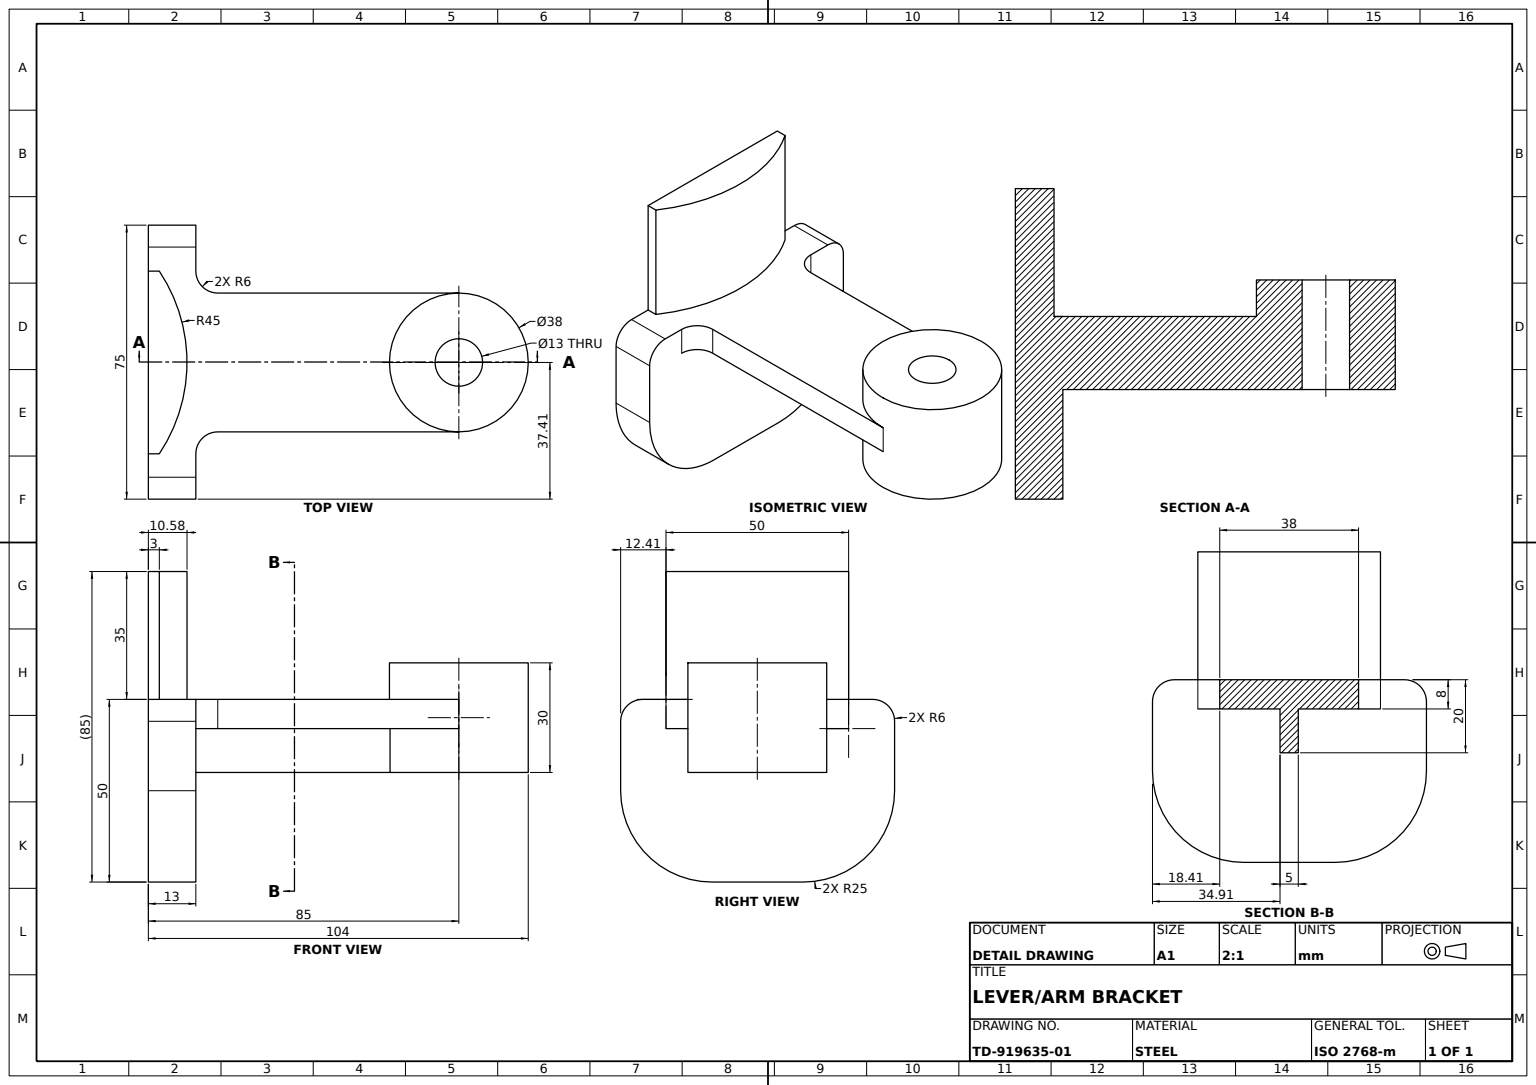
ISO-10303-21;
HEADER;
FILE_DESCRIPTION((''),'2;1');
FILE_NAME('','',(''),(''),'','','');
FILE_SCHEMA(('AUTOMOTIVE_DESIGN'));
ENDSEC;
DATA;
#1=APPLICATION_CONTEXT('');
#2=PRODUCT_CONTEXT('',#1,'mechanical');
#3=PRODUCT('','','',(#2));
#4=PRODUCT_DEFINITION_FORMATION('','',#3);
#5=PRODUCT_DEFINITION_CONTEXT('',#1,'design');
#6=PRODUCT_DEFINITION('','',#4,#5);
#7=PRODUCT_DEFINITION_SHAPE('','',#6);
#8=(LENGTH_UNIT()NAMED_UNIT(*)SI_UNIT(.MILLI.,.METRE.));
#9=(NAMED_UNIT(*)PLANE_ANGLE_UNIT()SI_UNIT($,.RADIAN.));
#10=(NAMED_UNIT(*)SI_UNIT($,.STERADIAN.)SOLID_ANGLE_UNIT());
#11=UNCERTAINTY_MEASURE_WITH_UNIT(LENGTH_MEASURE(1.E-05),#8,'distance_accuracy_value','');
#12=(GEOMETRIC_REPRESENTATION_CONTEXT(3)GLOBAL_UNCERTAINTY_ASSIGNED_CONTEXT((#11))GLOBAL_UNIT_ASSIGNED_CONTEXT((#8,#9,#10))REPRESENTATION_CONTEXT('',''));
#13=CARTESIAN_POINT('',(13.,42.,-34.91288));
#14=VERTEX_POINT('',#13);
#15=CARTESIAN_POINT('',(13.,30.,-34.91288));
#16=VERTEX_POINT('',#15);
#17=CARTESIAN_POINT('',(13.,0.,-34.91288));
#18=DIRECTION('',(0.,-1.,0.));
#19=VECTOR('',#18,1000.);
#20=LINE('',#17,#19);
#21=EDGE_CURVE('',#14,#16,#20,.T.);
#22=ORIENTED_EDGE('',*,*,#21,.T.);
#23=CARTESIAN_POINT('',(66.165192,30.,-34.91288));
#24=VERTEX_POINT('',#23);
#25=CARTESIAN_POINT('',(0.,30.,-34.91288));
#26=DIRECTION('',(1.,0.,0.));
#27=VECTOR('',#26,1000.);
#28=LINE('',#25,#27);
#29=EDGE_CURVE('',#16,#24,#28,.T.);
#30=ORIENTED_EDGE('',*,*,#29,.T.);
#31=CARTESIAN_POINT('',(66.165192,42.,-34.91288));
#32=VERTEX_POINT('',#31);
#33=DIRECTION('',(0.,1.,0.));
#34=VECTOR('',#33,1000.);
#35=LINE('',#23,#34);
#36=EDGE_CURVE('',#24,#32,#35,.T.);
#37=ORIENTED_EDGE('',*,*,#36,.T.);
#38=CARTESIAN_POINT('',(85.,42.,-34.91288));
#39=LINE('',#38,#27);
#40=EDGE_CURVE('',#14,#32,#39,.T.);
#41=ORIENTED_EDGE('',*,*,#40,.F.);
#42=EDGE_LOOP('',(#22,#30,#37,#41));
#43=FACE_OUTER_BOUND('',#42,.T.);
#44=DIRECTION('',(0.,0.,1.));
#45=AXIS2_PLACEMENT_3D('',#25,#44,#26);
#46=PLANE('',#45);
#47=ADVANCED_FACE('',(#43),#46,.T.);
#48=CARTESIAN_POINT('',(3.,85.,-12.41288));
#49=VERTEX_POINT('',#48);
#50=CARTESIAN_POINT('',(3.,50.,-12.41288));
#51=VERTEX_POINT('',#50);
#52=LINE('',#48,#19);
#53=EDGE_CURVE('',#49,#51,#52,.T.);
#54=ORIENTED_EDGE('',*,*,#53,.T.);
#55=CARTESIAN_POINT('',(3.,50.,-62.41288));
#56=VERTEX_POINT('',#55);
#57=CARTESIAN_POINT('',(-34.416574,50.,-37.41288));
#58=AXIS2_PLACEMENT_3D('',#57,#33,#44);
#59=CIRCLE('',#58,45.);
#60=EDGE_CURVE('',#51,#56,#59,.T.);
#61=ORIENTED_EDGE('',*,*,#60,.T.);
#62=CARTESIAN_POINT('',(3.,85.,-62.41288));
#63=VERTEX_POINT('',#62);
#64=LINE('',#62,#19);
#65=EDGE_CURVE('',#63,#56,#64,.T.);
#66=ORIENTED_EDGE('',*,*,#65,.F.);
#67=CARTESIAN_POINT('',(-34.416574,85.,-37.41288));
#68=AXIS2_PLACEMENT_3D('',#67,#33,#44);
#69=CIRCLE('',#68,45.);
#70=EDGE_CURVE('',#49,#63,#69,.T.);
#71=ORIENTED_EDGE('',*,*,#70,.F.);
#72=EDGE_LOOP('',(#54,#61,#66,#71));
#73=FACE_OUTER_BOUND('',#72,.T.);
#74=DIRECTION('',(0.,0.,-1.));
#75=AXIS2_PLACEMENT_3D('',#67,#18,#74);
#76=CYLINDRICAL_SURFACE('',#75,45.);
#77=ADVANCED_FACE('',(#73),#76,.T.);
#78=CARTESIAN_POINT('',(19.,50.,-18.41288));
#79=VERTEX_POINT('',#78);
#80=CARTESIAN_POINT('',(19.,42.,-18.41288));
#81=VERTEX_POINT('',#80);
#82=LINE('',#80,#19);
#83=EDGE_CURVE('',#79,#81,#82,.T.);
#84=ORIENTED_EDGE('',*,*,#83,.T.);
#85=CARTESIAN_POINT('',(85.,42.,-18.41288));
#86=VERTEX_POINT('',#85);
#87=LINE('',#85,#27);
#88=EDGE_CURVE('',#81,#86,#87,.T.);
#89=ORIENTED_EDGE('',*,*,#88,.T.);
#90=CARTESIAN_POINT('',(85.,50.,-18.41288));
#91=VERTEX_POINT('',#90);
#92=LINE('',#85,#34);
#93=EDGE_CURVE('',#86,#91,#92,.T.);
#94=ORIENTED_EDGE('',*,*,#93,.T.);
#95=LINE('',#90,#27);
#96=EDGE_CURVE('',#79,#91,#95,.T.);
#97=ORIENTED_EDGE('',*,*,#96,.F.);
#98=EDGE_LOOP('',(#84,#89,#94,#97));
#99=FACE_OUTER_BOUND('',#98,.T.);
#100=AXIS2_PLACEMENT_3D('',#85,#44,#26);
#101=PLANE('',#100);
#102=ADVANCED_FACE('',(#99),#101,.T.);
#103=CARTESIAN_POINT('',(85.,60.,-56.41288));
#104=VERTEX_POINT('',#103);
#105=CARTESIAN_POINT('',(85.,60.,-18.41288));
#106=VERTEX_POINT('',#105);
#107=CARTESIAN_POINT('',(85.,60.,-37.41288));
#108=AXIS2_PLACEMENT_3D('',#107,#33,#44);
#109=CIRCLE('',#108,19.);
#110=EDGE_CURVE('',#104,#106,#109,.T.);
#111=ORIENTED_EDGE('',*,*,#110,.F.);
#112=CARTESIAN_POINT('',(85.,50.,-56.41288));
#113=VERTEX_POINT('',#112);
#114=LINE('',#103,#19);
#115=EDGE_CURVE('',#104,#113,#114,.T.);
#116=ORIENTED_EDGE('',*,*,#115,.T.);
#117=CARTESIAN_POINT('',(85.,50.,-37.41288));
#118=AXIS2_PLACEMENT_3D('',#117,#18,#44);
#119=CIRCLE('',#118,19.);
#120=EDGE_CURVE('',#91,#113,#119,.T.);
#121=ORIENTED_EDGE('',*,*,#120,.F.);
#122=LINE('',#105,#19);
#123=EDGE_CURVE('',#106,#91,#122,.T.);
#124=ORIENTED_EDGE('',*,*,#123,.F.);
#125=EDGE_LOOP('',(#111,#116,#121,#124));
#126=FACE_OUTER_BOUND('',#125,.T.);
#127=AXIS2_PLACEMENT_3D('',#107,#18,#74);
#128=CYLINDRICAL_SURFACE('',#127,19.);
#129=ADVANCED_FACE('',(#126),#128,.T.);
#130=CARTESIAN_POINT('',(0.,0.,-50.));
#131=VERTEX_POINT('',#130);
#132=CARTESIAN_POINT('',(0.,0.,-25.));
#133=VERTEX_POINT('',#132);
#134=CARTESIAN_POINT('',(0.,0.,-75.));
#135=VECTOR('',#44,1000.);
#136=LINE('',#134,#135);
#137=EDGE_CURVE('',#131,#133,#136,.T.);
#138=ORIENTED_EDGE('',*,*,#137,.F.);
#139=CARTESIAN_POINT('',(13.,0.,-50.));
#140=VERTEX_POINT('',#139);
#141=LINE('',#130,#27);
#142=EDGE_CURVE('',#131,#140,#141,.T.);
#143=ORIENTED_EDGE('',*,*,#142,.T.);
#144=CARTESIAN_POINT('',(13.,0.,-25.));
#145=VERTEX_POINT('',#144);
#146=CARTESIAN_POINT('',(13.,0.,-75.));
#147=LINE('',#146,#135);
#148=EDGE_CURVE('',#140,#145,#147,.T.);
#149=ORIENTED_EDGE('',*,*,#148,.T.);
#150=DIRECTION('',(-1.,0.,0.));
#151=VECTOR('',#150,1000.);
#152=LINE('',#132,#151);
#153=EDGE_CURVE('',#145,#133,#152,.T.);
#154=ORIENTED_EDGE('',*,*,#153,.T.);
#155=EDGE_LOOP('',(#138,#143,#149,#154));
#156=FACE_OUTER_BOUND('',#155,.T.);
#157=AXIS2_PLACEMENT_3D('',#134,#18,#74);
#158=PLANE('',#157);
#159=ADVANCED_FACE('',(#156),#158,.T.);
#160=CARTESIAN_POINT('',(13.,30.,-39.91288));
#161=VERTEX_POINT('',#160);
#162=CARTESIAN_POINT('',(13.,42.,-39.91288));
#163=VERTEX_POINT('',#162);
#164=CARTESIAN_POINT('',(13.,0.,-39.91288));
#165=LINE('',#164,#34);
#166=EDGE_CURVE('',#161,#163,#165,.T.);
#167=ORIENTED_EDGE('',*,*,#166,.T.);
#168=CARTESIAN_POINT('',(66.165192,42.,-39.91288));
#169=VERTEX_POINT('',#168);
#170=CARTESIAN_POINT('',(85.,42.,-39.91288));
#171=LINE('',#170,#151);
#172=EDGE_CURVE('',#169,#163,#171,.T.);
#173=ORIENTED_EDGE('',*,*,#172,.F.);
#174=CARTESIAN_POINT('',(66.165192,30.,-39.91288));
#175=VERTEX_POINT('',#174);
#176=LINE('',#174,#34);
#177=EDGE_CURVE('',#175,#169,#176,.T.);
#178=ORIENTED_EDGE('',*,*,#177,.F.);
#179=CARTESIAN_POINT('',(0.,30.,-39.91288));
#180=LINE('',#179,#151);
#181=EDGE_CURVE('',#175,#161,#180,.T.);
#182=ORIENTED_EDGE('',*,*,#181,.T.);
#183=EDGE_LOOP('',(#167,#173,#178,#182));
#184=FACE_OUTER_BOUND('',#183,.T.);
#185=AXIS2_PLACEMENT_3D('',#179,#74,#150);
#186=PLANE('',#185);
#187=ADVANCED_FACE('',(#184),#186,.T.);
#188=CARTESIAN_POINT('',(0.,25.,0.));
#189=VERTEX_POINT('',#188);
#190=CARTESIAN_POINT('',(0.,25.,-25.));
#191=AXIS2_PLACEMENT_3D('',#190,#150,#44);
#192=CIRCLE('',#191,25.);
#193=EDGE_CURVE('',#133,#189,#192,.T.);
#194=ORIENTED_EDGE('',*,*,#193,.T.);
#195=CARTESIAN_POINT('',(0.,44.,0.));
#196=VERTEX_POINT('',#195);
#197=CARTESIAN_POINT('',(0.,0.,0.));
#198=LINE('',#197,#19);
#199=EDGE_CURVE('',#196,#189,#198,.T.);
#200=ORIENTED_EDGE('',*,*,#199,.F.);
#201=CARTESIAN_POINT('',(0.,50.,-6.));
#202=VERTEX_POINT('',#201);
#203=CARTESIAN_POINT('',(0.,44.,-6.));
#204=AXIS2_PLACEMENT_3D('',#203,#150,#44);
#205=CIRCLE('',#204,6.);
#206=EDGE_CURVE('',#196,#202,#205,.T.);
#207=ORIENTED_EDGE('',*,*,#206,.T.);
#208=CARTESIAN_POINT('',(0.,50.,-12.41288));
#209=VERTEX_POINT('',#208);
#210=CARTESIAN_POINT('',(0.,50.,-75.));
#211=LINE('',#210,#135);
#212=EDGE_CURVE('',#209,#202,#211,.T.);
#213=ORIENTED_EDGE('',*,*,#212,.F.);
#214=CARTESIAN_POINT('',(0.,85.,-12.41288));
#215=VERTEX_POINT('',#214);
#216=LINE('',#214,#19);
#217=EDGE_CURVE('',#215,#209,#216,.T.);
#218=ORIENTED_EDGE('',*,*,#217,.F.);
#219=CARTESIAN_POINT('',(0.,85.,-62.41288));
#220=VERTEX_POINT('',#219);
#221=CARTESIAN_POINT('',(0.,85.,0.));
#222=LINE('',#221,#135);
#223=EDGE_CURVE('',#220,#215,#222,.T.);
#224=ORIENTED_EDGE('',*,*,#223,.F.);
#225=CARTESIAN_POINT('',(0.,50.,-62.41288));
#226=VERTEX_POINT('',#225);
#227=LINE('',#219,#19);
#228=EDGE_CURVE('',#220,#226,#227,.T.);
#229=ORIENTED_EDGE('',*,*,#228,.T.);
#230=CARTESIAN_POINT('',(0.,50.,-69.));
#231=VERTEX_POINT('',#230);
#232=EDGE_CURVE('',#231,#226,#211,.T.);
#233=ORIENTED_EDGE('',*,*,#232,.F.);
#234=CARTESIAN_POINT('',(0.,44.,-75.));
#235=VERTEX_POINT('',#234);
#236=CARTESIAN_POINT('',(0.,44.,-69.));
#237=AXIS2_PLACEMENT_3D('',#236,#150,#44);
#238=CIRCLE('',#237,6.);
#239=EDGE_CURVE('',#231,#235,#238,.T.);
#240=ORIENTED_EDGE('',*,*,#239,.T.);
#241=CARTESIAN_POINT('',(0.,25.,-75.));
#242=VERTEX_POINT('',#241);
#243=LINE('',#134,#19);
#244=EDGE_CURVE('',#235,#242,#243,.T.);
#245=ORIENTED_EDGE('',*,*,#244,.T.);
#246=CARTESIAN_POINT('',(0.,25.,-50.));
#247=AXIS2_PLACEMENT_3D('',#246,#150,#44);
#248=CIRCLE('',#247,25.);
#249=EDGE_CURVE('',#242,#131,#248,.T.);
#250=ORIENTED_EDGE('',*,*,#249,.T.);
#251=ORIENTED_EDGE('',*,*,#137,.T.);
#252=EDGE_LOOP('',(#194,#200,#207,#213,#218,#224,#229,#233,#240,#245,#250,#251));
#253=FACE_OUTER_BOUND('',#252,.T.);
#254=AXIS2_PLACEMENT_3D('',#134,#150,#44);
#255=PLANE('',#254);
#256=ADVANCED_FACE('',(#253),#255,.T.);
#257=ORIENTED_EDGE('',*,*,#172,.T.);
#258=CARTESIAN_POINT('',(13.,42.,-62.41288));
#259=VERTEX_POINT('',#258);
#260=CARTESIAN_POINT('',(13.,42.,-56.41288));
#261=LINE('',#260,#135);
#262=EDGE_CURVE('',#259,#163,#261,.T.);
#263=ORIENTED_EDGE('',*,*,#262,.F.);
#264=CARTESIAN_POINT('',(19.,42.,-56.41288));
#265=VERTEX_POINT('',#264);
#266=CARTESIAN_POINT('',(19.,42.,-62.41288));
#267=AXIS2_PLACEMENT_3D('',#266,#33,#44);
#268=CIRCLE('',#267,6.);
#269=EDGE_CURVE('',#259,#265,#268,.T.);
#270=ORIENTED_EDGE('',*,*,#269,.T.);
#271=CARTESIAN_POINT('',(85.,42.,-56.41288));
#272=VERTEX_POINT('',#271);
#273=LINE('',#271,#151);
#274=EDGE_CURVE('',#272,#265,#273,.T.);
#275=ORIENTED_EDGE('',*,*,#274,.F.);
#276=CARTESIAN_POINT('',(85.,42.,-37.41288));
#277=AXIS2_PLACEMENT_3D('',#276,#18,#44);
#278=CIRCLE('',#277,19.);
#279=EDGE_CURVE('',#169,#272,#278,.T.);
#280=ORIENTED_EDGE('',*,*,#279,.F.);
#281=EDGE_LOOP('',(#257,#263,#270,#275,#280));
#282=FACE_OUTER_BOUND('',#281,.T.);
#283=AXIS2_PLACEMENT_3D('',#276,#33,#44);
#284=PLANE('',#283);
#285=ADVANCED_FACE('',(#282),#284,.F.);
#286=ORIENTED_EDGE('',*,*,#177,.T.);
#287=ORIENTED_EDGE('',*,*,#279,.T.);
#288=CARTESIAN_POINT('',(85.,30.,-56.41288));
#289=VERTEX_POINT('',#288);
#290=EDGE_CURVE('',#272,#289,#114,.T.);
#291=ORIENTED_EDGE('',*,*,#290,.T.);
#292=CARTESIAN_POINT('',(85.,30.,-37.41288));
#293=AXIS2_PLACEMENT_3D('',#292,#33,#44);
#294=CIRCLE('',#293,19.);
#295=EDGE_CURVE('',#289,#175,#294,.T.);
#296=ORIENTED_EDGE('',*,*,#295,.T.);
#297=EDGE_LOOP('',(#286,#287,#291,#296));
#298=FACE_OUTER_BOUND('',#297,.T.);
#299=ADVANCED_FACE('',(#298),#128,.T.);
#300=CARTESIAN_POINT('',(13.,44.,-75.));
#301=VERTEX_POINT('',#300);
#302=LINE('',#234,#27);
#303=EDGE_CURVE('',#235,#301,#302,.T.);
#304=ORIENTED_EDGE('',*,*,#303,.F.);
#305=ORIENTED_EDGE('',*,*,#239,.F.);
#306=CARTESIAN_POINT('',(13.,50.,-69.));
#307=VERTEX_POINT('',#306);
#308=LINE('',#230,#151);
#309=EDGE_CURVE('',#307,#231,#308,.T.);
#310=ORIENTED_EDGE('',*,*,#309,.F.);
#311=CARTESIAN_POINT('',(13.,44.,-69.));
#312=AXIS2_PLACEMENT_3D('',#311,#26,#74);
#313=CIRCLE('',#312,6.);
#314=EDGE_CURVE('',#301,#307,#313,.T.);
#315=ORIENTED_EDGE('',*,*,#314,.F.);
#316=EDGE_LOOP('',(#304,#305,#310,#315));
#317=FACE_OUTER_BOUND('',#316,.T.);
#318=CYLINDRICAL_SURFACE('',#237,6.);
#319=ADVANCED_FACE('',(#317),#318,.T.);
#320=CARTESIAN_POINT('',(85.,30.,-18.41288));
#321=VERTEX_POINT('',#320);
#322=EDGE_CURVE('',#321,#289,#294,.T.);
#323=ORIENTED_EDGE('',*,*,#322,.T.);
#324=ORIENTED_EDGE('',*,*,#290,.F.);
#325=LINE('',#271,#34);
#326=EDGE_CURVE('',#272,#113,#325,.T.);
#327=ORIENTED_EDGE('',*,*,#326,.T.);
#328=ORIENTED_EDGE('',*,*,#115,.F.);
#329=EDGE_CURVE('',#106,#104,#109,.T.);
#330=ORIENTED_EDGE('',*,*,#329,.F.);
#331=ORIENTED_EDGE('',*,*,#123,.T.);
#332=ORIENTED_EDGE('',*,*,#93,.F.);
#333=EDGE_CURVE('',#86,#321,#122,.T.);
#334=ORIENTED_EDGE('',*,*,#333,.T.);
#335=EDGE_LOOP('',(#323,#324,#327,#328,#330,#331,#332,#334));
#336=FACE_OUTER_BOUND('',#335,.T.);
#337=ADVANCED_FACE('',(#336),#128,.T.);
#338=ORIENTED_EDGE('',*,*,#60,.F.);
#339=LINE('',#208,#27);
#340=EDGE_CURVE('',#209,#51,#339,.T.);
#341=ORIENTED_EDGE('',*,*,#340,.F.);
#342=ORIENTED_EDGE('',*,*,#212,.T.);
#343=CARTESIAN_POINT('',(13.,50.,-6.));
#344=VERTEX_POINT('',#343);
#345=LINE('',#343,#27);
#346=EDGE_CURVE('',#202,#344,#345,.T.);
#347=ORIENTED_EDGE('',*,*,#346,.T.);
#348=CARTESIAN_POINT('',(13.,50.,-12.41288));
#349=VERTEX_POINT('',#348);
#350=CARTESIAN_POINT('',(13.,50.,-75.));
#351=LINE('',#350,#135);
#352=EDGE_CURVE('',#349,#344,#351,.T.);
#353=ORIENTED_EDGE('',*,*,#352,.F.);
#354=CARTESIAN_POINT('',(19.,50.,-12.41288));
#355=AXIS2_PLACEMENT_3D('',#354,#18,#44);
#356=CIRCLE('',#355,6.);
#357=EDGE_CURVE('',#349,#79,#356,.T.);
#358=ORIENTED_EDGE('',*,*,#357,.T.);
#359=ORIENTED_EDGE('',*,*,#96,.T.);
#360=ORIENTED_EDGE('',*,*,#120,.T.);
#361=CARTESIAN_POINT('',(19.,50.,-56.41288));
#362=VERTEX_POINT('',#361);
#363=LINE('',#112,#151);
#364=EDGE_CURVE('',#113,#362,#363,.T.);
#365=ORIENTED_EDGE('',*,*,#364,.T.);
#366=CARTESIAN_POINT('',(13.,50.,-62.41288));
#367=VERTEX_POINT('',#366);
#368=CARTESIAN_POINT('',(19.,50.,-62.41288));
#369=AXIS2_PLACEMENT_3D('',#368,#18,#44);
#370=CIRCLE('',#369,6.);
#371=EDGE_CURVE('',#362,#367,#370,.T.);
#372=ORIENTED_EDGE('',*,*,#371,.T.);
#373=EDGE_CURVE('',#307,#367,#351,.T.);
#374=ORIENTED_EDGE('',*,*,#373,.F.);
#375=ORIENTED_EDGE('',*,*,#309,.T.);
#376=ORIENTED_EDGE('',*,*,#232,.T.);
#377=LINE('',#225,#27);
#378=EDGE_CURVE('',#226,#56,#377,.T.);
#379=ORIENTED_EDGE('',*,*,#378,.T.);
#380=EDGE_LOOP('',(#338,#341,#342,#347,#353,#358,#359,#360,#365,#372,#374,#375,#376,#379));
#381=FACE_OUTER_BOUND('',#380,.T.);
#382=AXIS2_PLACEMENT_3D('',#210,#33,#44);
#383=PLANE('',#382);
#384=ADVANCED_FACE('',(#381),#383,.T.);
#385=CARTESIAN_POINT('',(13.,25.,0.));
#386=VERTEX_POINT('',#385);
#387=CARTESIAN_POINT('',(13.,25.,-25.));
#388=AXIS2_PLACEMENT_3D('',#387,#26,#74);
#389=CIRCLE('',#388,25.);
#390=EDGE_CURVE('',#386,#145,#389,.T.);
#391=ORIENTED_EDGE('',*,*,#390,.F.);
#392=LINE('',#385,#27);
#393=EDGE_CURVE('',#189,#386,#392,.T.);
#394=ORIENTED_EDGE('',*,*,#393,.F.);
#395=ORIENTED_EDGE('',*,*,#193,.F.);
#396=ORIENTED_EDGE('',*,*,#153,.F.);
#397=EDGE_LOOP('',(#391,#394,#395,#396));
#398=FACE_OUTER_BOUND('',#397,.T.);
#399=CYLINDRICAL_SURFACE('',#191,25.);
#400=ADVANCED_FACE('',(#398),#399,.T.);
#401=CARTESIAN_POINT('',(13.,42.,-12.41288));
#402=VERTEX_POINT('',#401);
#403=CARTESIAN_POINT('',(19.,42.,-12.41288));
#404=AXIS2_PLACEMENT_3D('',#403,#33,#44);
#405=CIRCLE('',#404,6.);
#406=EDGE_CURVE('',#81,#402,#405,.T.);
#407=ORIENTED_EDGE('',*,*,#406,.F.);
#408=ORIENTED_EDGE('',*,*,#83,.F.);
#409=ORIENTED_EDGE('',*,*,#357,.F.);
#410=LINE('',#348,#34);
#411=EDGE_CURVE('',#402,#349,#410,.T.);
#412=ORIENTED_EDGE('',*,*,#411,.F.);
#413=EDGE_LOOP('',(#407,#408,#409,#412));
#414=FACE_OUTER_BOUND('',#413,.T.);
#415=CARTESIAN_POINT('',(19.,0.,-12.41288));
#416=AXIS2_PLACEMENT_3D('',#415,#18,#74);
#417=CYLINDRICAL_SURFACE('',#416,6.);
#418=ADVANCED_FACE('',(#414),#417,.F.);
#419=ORIENTED_EDGE('',*,*,#40,.T.);
#420=EDGE_CURVE('',#86,#32,#278,.T.);
#421=ORIENTED_EDGE('',*,*,#420,.F.);
#422=ORIENTED_EDGE('',*,*,#88,.F.);
#423=ORIENTED_EDGE('',*,*,#406,.T.);
#424=EDGE_CURVE('',#14,#402,#261,.T.);
#425=ORIENTED_EDGE('',*,*,#424,.F.);
#426=EDGE_LOOP('',(#419,#421,#422,#423,#425));
#427=FACE_OUTER_BOUND('',#426,.T.);
#428=ADVANCED_FACE('',(#427),#284,.F.);
#429=CARTESIAN_POINT('',(13.,44.,0.));
#430=VERTEX_POINT('',#429);
#431=CARTESIAN_POINT('',(13.,0.,0.));
#432=LINE('',#431,#34);
#433=EDGE_CURVE('',#386,#430,#432,.T.);
#434=ORIENTED_EDGE('',*,*,#433,.F.);
#435=ORIENTED_EDGE('',*,*,#390,.T.);
#436=ORIENTED_EDGE('',*,*,#148,.F.);
#437=CARTESIAN_POINT('',(13.,25.,-75.));
#438=VERTEX_POINT('',#437);
#439=CARTESIAN_POINT('',(13.,25.,-50.));
#440=AXIS2_PLACEMENT_3D('',#439,#26,#74);
#441=CIRCLE('',#440,25.);
#442=EDGE_CURVE('',#140,#438,#441,.T.);
#443=ORIENTED_EDGE('',*,*,#442,.T.);
#444=LINE('',#146,#34);
#445=EDGE_CURVE('',#438,#301,#444,.T.);
#446=ORIENTED_EDGE('',*,*,#445,.T.);
#447=ORIENTED_EDGE('',*,*,#314,.T.);
#448=ORIENTED_EDGE('',*,*,#373,.T.);
#449=LINE('',#258,#19);
#450=EDGE_CURVE('',#367,#259,#449,.T.);
#451=ORIENTED_EDGE('',*,*,#450,.T.);
#452=ORIENTED_EDGE('',*,*,#262,.T.);
#453=ORIENTED_EDGE('',*,*,#166,.F.);
#454=CARTESIAN_POINT('',(13.,30.,-75.));
#455=LINE('',#454,#135);
#456=EDGE_CURVE('',#161,#16,#455,.T.);
#457=ORIENTED_EDGE('',*,*,#456,.T.);
#458=ORIENTED_EDGE('',*,*,#21,.F.);
#459=ORIENTED_EDGE('',*,*,#424,.T.);
#460=ORIENTED_EDGE('',*,*,#411,.T.);
#461=ORIENTED_EDGE('',*,*,#352,.T.);
#462=CARTESIAN_POINT('',(13.,44.,-6.));
#463=AXIS2_PLACEMENT_3D('',#462,#26,#74);
#464=CIRCLE('',#463,6.);
#465=EDGE_CURVE('',#344,#430,#464,.T.);
#466=ORIENTED_EDGE('',*,*,#465,.T.);
#467=EDGE_LOOP('',(#434,#435,#436,#443,#446,#447,#448,#451,#452,#453,#457,#458,#459,#460,#461,#466));
#468=FACE_OUTER_BOUND('',#467,.T.);
#469=AXIS2_PLACEMENT_3D('',#146,#26,#74);
#470=PLANE('',#469);
#471=ADVANCED_FACE('',(#468),#470,.T.);
#472=CARTESIAN_POINT('',(85.,30.,-30.91288));
#473=VERTEX_POINT('',#472);
#474=CARTESIAN_POINT('',(85.,30.,-43.91288));
#475=VERTEX_POINT('',#474);
#476=CIRCLE('',#293,6.5);
#477=EDGE_CURVE('',#473,#475,#476,.T.);
#478=ORIENTED_EDGE('',*,*,#477,.T.);
#479=EDGE_CURVE('',#475,#473,#476,.T.);
#480=ORIENTED_EDGE('',*,*,#479,.T.);
#481=EDGE_LOOP('',(#478,#480));
#482=FACE_BOUND('',#481,.T.);
#483=ORIENTED_EDGE('',*,*,#181,.F.);
#484=ORIENTED_EDGE('',*,*,#295,.F.);
#485=ORIENTED_EDGE('',*,*,#322,.F.);
#486=EDGE_CURVE('',#24,#321,#294,.T.);
#487=ORIENTED_EDGE('',*,*,#486,.F.);
#488=ORIENTED_EDGE('',*,*,#29,.F.);
#489=ORIENTED_EDGE('',*,*,#456,.F.);
#490=EDGE_LOOP('',(#483,#484,#485,#487,#488,#489));
#491=FACE_OUTER_BOUND('',#490,.T.);
#492=CARTESIAN_POINT('',(0.,30.,0.));
#493=AXIS2_PLACEMENT_3D('',#492,#33,#44);
#494=PLANE('',#493);
#495=ADVANCED_FACE('',(#482,#491),#494,.F.);
#496=LINE('',#195,#151);
#497=EDGE_CURVE('',#430,#196,#496,.T.);
#498=ORIENTED_EDGE('',*,*,#497,.F.);
#499=ORIENTED_EDGE('',*,*,#465,.F.);
#500=ORIENTED_EDGE('',*,*,#346,.F.);
#501=ORIENTED_EDGE('',*,*,#206,.F.);
#502=EDGE_LOOP('',(#498,#499,#500,#501));
#503=FACE_OUTER_BOUND('',#502,.T.);
#504=AXIS2_PLACEMENT_3D('',#203,#26,#74);
#505=CYLINDRICAL_SURFACE('',#504,6.);
#506=ADVANCED_FACE('',(#503),#505,.T.);
#507=ORIENTED_EDGE('',*,*,#274,.T.);
#508=LINE('',#361,#34);
#509=EDGE_CURVE('',#265,#362,#508,.T.);
#510=ORIENTED_EDGE('',*,*,#509,.T.);
#511=ORIENTED_EDGE('',*,*,#364,.F.);
#512=ORIENTED_EDGE('',*,*,#326,.F.);
#513=EDGE_LOOP('',(#507,#510,#511,#512));
#514=FACE_OUTER_BOUND('',#513,.T.);
#515=AXIS2_PLACEMENT_3D('',#271,#74,#150);
#516=PLANE('',#515);
#517=ADVANCED_FACE('',(#514),#516,.T.);
#518=CARTESIAN_POINT('',(85.,60.,-43.91288));
#519=VERTEX_POINT('',#518);
#520=LINE('',#518,#19);
#521=EDGE_CURVE('',#519,#475,#520,.T.);
#522=ORIENTED_EDGE('',*,*,#521,.T.);
#523=ORIENTED_EDGE('',*,*,#477,.F.);
#524=CARTESIAN_POINT('',(85.,60.,-30.91288));
#525=VERTEX_POINT('',#524);
#526=LINE('',#524,#19);
#527=EDGE_CURVE('',#525,#473,#526,.T.);
#528=ORIENTED_EDGE('',*,*,#527,.F.);
#529=CIRCLE('',#108,6.5);
#530=EDGE_CURVE('',#525,#519,#529,.T.);
#531=ORIENTED_EDGE('',*,*,#530,.T.);
#532=EDGE_LOOP('',(#522,#523,#528,#531));
#533=FACE_OUTER_BOUND('',#532,.T.);
#534=CYLINDRICAL_SURFACE('',#127,6.5);
#535=ADVANCED_FACE('',(#533),#534,.F.);
#536=ORIENTED_EDGE('',*,*,#433,.T.);
#537=ORIENTED_EDGE('',*,*,#497,.T.);
#538=ORIENTED_EDGE('',*,*,#199,.T.);
#539=ORIENTED_EDGE('',*,*,#393,.T.);
#540=EDGE_LOOP('',(#536,#537,#538,#539));
#541=FACE_OUTER_BOUND('',#540,.T.);
#542=AXIS2_PLACEMENT_3D('',#197,#74,#150);
#543=PLANE('',#542);
#544=ADVANCED_FACE('',(#541),#543,.F.);
#545=ORIENTED_EDGE('',*,*,#527,.T.);
#546=ORIENTED_EDGE('',*,*,#479,.F.);
#547=ORIENTED_EDGE('',*,*,#521,.F.);
#548=EDGE_CURVE('',#519,#525,#529,.T.);
#549=ORIENTED_EDGE('',*,*,#548,.T.);
#550=EDGE_LOOP('',(#545,#546,#547,#549));
#551=FACE_OUTER_BOUND('',#550,.T.);
#552=ADVANCED_FACE('',(#551),#534,.F.);
#553=ORIENTED_EDGE('',*,*,#36,.F.);
#554=ORIENTED_EDGE('',*,*,#486,.T.);
#555=ORIENTED_EDGE('',*,*,#333,.F.);
#556=ORIENTED_EDGE('',*,*,#420,.T.);
#557=EDGE_LOOP('',(#553,#554,#555,#556));
#558=FACE_OUTER_BOUND('',#557,.T.);
#559=ADVANCED_FACE('',(#558),#128,.T.);
#560=ORIENTED_EDGE('',*,*,#269,.F.);
#561=ORIENTED_EDGE('',*,*,#450,.F.);
#562=ORIENTED_EDGE('',*,*,#371,.F.);
#563=ORIENTED_EDGE('',*,*,#509,.F.);
#564=EDGE_LOOP('',(#560,#561,#562,#563));
#565=FACE_OUTER_BOUND('',#564,.T.);
#566=AXIS2_PLACEMENT_3D('',#266,#18,#74);
#567=CYLINDRICAL_SURFACE('',#566,6.);
#568=ADVANCED_FACE('',(#565),#567,.F.);
#569=ORIENTED_EDGE('',*,*,#442,.F.);
#570=ORIENTED_EDGE('',*,*,#142,.F.);
#571=ORIENTED_EDGE('',*,*,#249,.F.);
#572=LINE('',#241,#151);
#573=EDGE_CURVE('',#438,#242,#572,.T.);
#574=ORIENTED_EDGE('',*,*,#573,.F.);
#575=EDGE_LOOP('',(#569,#570,#571,#574));
#576=FACE_OUTER_BOUND('',#575,.T.);
#577=AXIS2_PLACEMENT_3D('',#246,#26,#74);
#578=CYLINDRICAL_SURFACE('',#577,25.);
#579=ADVANCED_FACE('',(#576),#578,.T.);
#580=ORIENTED_EDGE('',*,*,#244,.F.);
#581=ORIENTED_EDGE('',*,*,#303,.T.);
#582=ORIENTED_EDGE('',*,*,#445,.F.);
#583=ORIENTED_EDGE('',*,*,#573,.T.);
#584=EDGE_LOOP('',(#580,#581,#582,#583));
#585=FACE_OUTER_BOUND('',#584,.T.);
#586=AXIS2_PLACEMENT_3D('',#134,#74,#150);
#587=PLANE('',#586);
#588=ADVANCED_FACE('',(#585),#587,.T.);
#589=LINE('',#219,#27);
#590=EDGE_CURVE('',#220,#63,#589,.T.);
#591=ORIENTED_EDGE('',*,*,#590,.T.);
#592=ORIENTED_EDGE('',*,*,#65,.T.);
#593=ORIENTED_EDGE('',*,*,#378,.F.);
#594=ORIENTED_EDGE('',*,*,#228,.F.);
#595=EDGE_LOOP('',(#591,#592,#593,#594));
#596=FACE_OUTER_BOUND('',#595,.T.);
#597=AXIS2_PLACEMENT_3D('',#219,#74,#150);
#598=PLANE('',#597);
#599=ADVANCED_FACE('',(#596),#598,.T.);
#600=LINE('',#214,#27);
#601=EDGE_CURVE('',#215,#49,#600,.T.);
#602=ORIENTED_EDGE('',*,*,#601,.F.);
#603=ORIENTED_EDGE('',*,*,#217,.T.);
#604=ORIENTED_EDGE('',*,*,#340,.T.);
#605=ORIENTED_EDGE('',*,*,#53,.F.);
#606=EDGE_LOOP('',(#602,#603,#604,#605));
#607=FACE_OUTER_BOUND('',#606,.T.);
#608=AXIS2_PLACEMENT_3D('',#214,#74,#150);
#609=PLANE('',#608);
#610=ADVANCED_FACE('',(#607),#609,.F.);
#611=ORIENTED_EDGE('',*,*,#601,.T.);
#612=ORIENTED_EDGE('',*,*,#70,.T.);
#613=ORIENTED_EDGE('',*,*,#590,.F.);
#614=ORIENTED_EDGE('',*,*,#223,.T.);
#615=EDGE_LOOP('',(#611,#612,#613,#614));
#616=FACE_OUTER_BOUND('',#615,.T.);
#617=AXIS2_PLACEMENT_3D('',#221,#33,#44);
#618=PLANE('',#617);
#619=ADVANCED_FACE('',(#616),#618,.T.);
#620=ORIENTED_EDGE('',*,*,#329,.T.);
#621=ORIENTED_EDGE('',*,*,#110,.T.);
#622=EDGE_LOOP('',(#620,#621));
#623=FACE_OUTER_BOUND('',#622,.T.);
#624=ORIENTED_EDGE('',*,*,#530,.F.);
#625=ORIENTED_EDGE('',*,*,#548,.F.);
#626=EDGE_LOOP('',(#624,#625));
#627=FACE_BOUND('',#626,.T.);
#628=CARTESIAN_POINT('',(0.,60.,0.));
#629=AXIS2_PLACEMENT_3D('',#628,#33,#44);
#630=PLANE('',#629);
#631=ADVANCED_FACE('',(#623,#627),#630,.T.);
#632=CLOSED_SHELL('',(#47,#77,#102,#129,#159,#187,#256,#285,#299,#319,#337,#384,#400,#418,#428,#471,#495,#506,#517,#535,#544,#552,#559,#568,#579,#588,#599,#610,#619,#631));
#633=MANIFOLD_SOLID_BREP('',#632);
#634=ADVANCED_BREP_SHAPE_REPRESENTATION('',(#633),#12);
#635=SHAPE_DEFINITION_REPRESENTATION(#7,#634);
ENDSEC;
END-ISO-10303-21;
